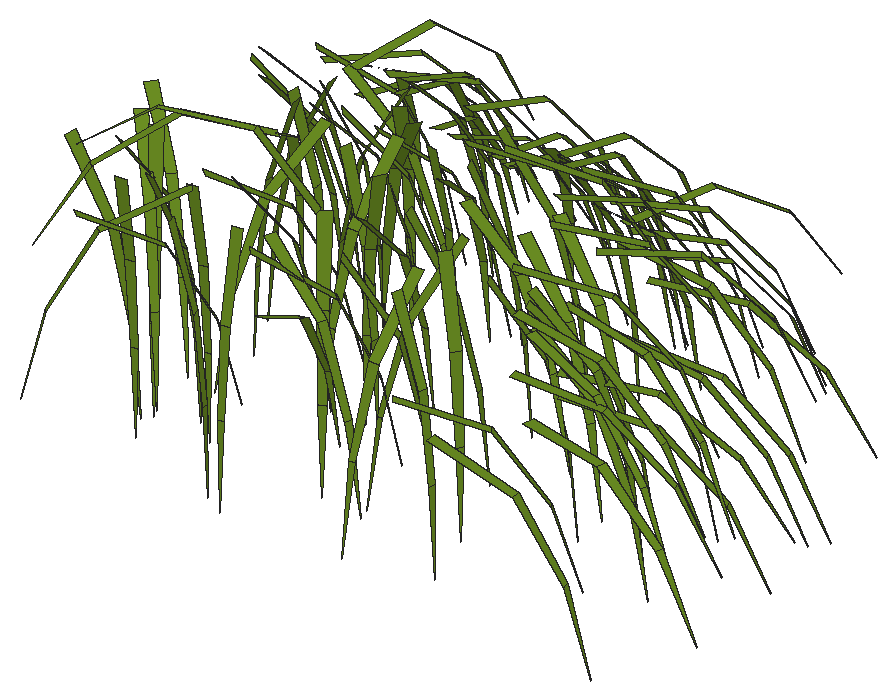
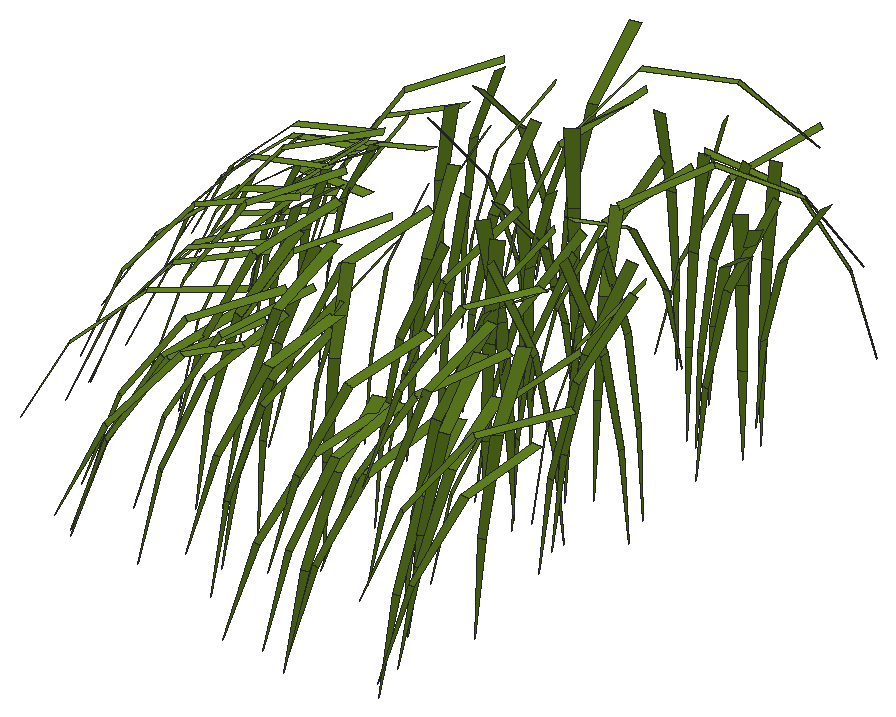
# SketchUp Ruby script. Lengths in inches.
U = 1.inch
M = Sketchup.active_model
def pt(a) = Geom::Point3d.new(a.map { |v| v * U })
def face(e, loops, mat)
  f = e.add_face(loops[0].map { |a| pt(a) })
  loops[1..].each { |l| e.add_face(l.map { |a| pt(a) }).erase! }
  f.material = f.back_material = mat if mat
  f
end
# faces: each face lists its corners as indices into pts; further lists are holes
def faces(e, pts, list, mat = nil) = list.each { |f| face(e, (f[0].is_a?(Array) ? f : [f]).map { |l| l.map { |i| pts[i] } }, mat) }
# xy, xz, yz: faces in a plane at the given z, y or x. An outline is a flat list of corners, or four numbers for a rectangle; further outlines are holes
def ring(l) = l.size == 4 ? [[l[0], l[1]], [l[2], l[1]], [l[2], l[3]], [l[0], l[3]]] : l.each_slice(2).to_a
def flat(e, list, mat, &to3) = list.each { |f| face(e, (f[0].is_a?(Array) ? f : [f]).map { |l| ring(l).map { |u, v| to3.(u, v) } }, mat) }
def xy(e, z, list, mat = nil) = flat(e, list, mat) { |x, y| [x, y, z] }
def xz(e, y, list, mat = nil) = flat(e, list, mat) { |x, z| [x, y, z] }
def yz(e, x, list, mat = nil) = flat(e, list, mat) { |y, z| [x, y, z] }
def lines(e, pts, list) = list.each { |a, b| e.add_line(pt(pts[a]), pt(pts[b])) }
# prism: a flat outline (further loops are holes) pulled along v
def prism(e, loops, v, mat = nil)
  f = face(e, loops, mat); d = Geom::Vector3d.new(v.map { |x| x * U })
  f.pushpull(f.normal.samedirection?(d) ? d.length : -d.length)
end
def box(e, o, s, mat = nil) = prism(e, [[o, [o[0] + s[0], o[1], o[2]], [o[0] + s[0], o[1] + s[1], o[2]], [o[0], o[1] + s[1], o[2]]]], [0, 0, s[2]], mat)
def at(x, y, z, deg = 0) = Geom::Transformation.translation(pt([x, y, z])) * Geom::Transformation.rotation(ORIGIN, Z_AXIS, deg.degrees)
def axes(o, x, y, z) = Geom::Transformation.new([*x, 0, *y, 0, *z, 0, *pt(o).to_a, 1])
def part(name) = M.definitions.add(name)
# library, detail: a bought-in or finely detailed component or shape, given as its bounding box
def library(name, o, s) = part(name).tap { |d| box(d.entities, o, s) }
def detail(e, o, s) = box(e.add_group.entities, o, s)
def put(e, d, t, mat = nil) = e.add_instance(d, t).tap { |i| i.material = mat if mat }
def group(e, t, mat = nil) = e.add_group.tap { |g| g.transformation = t; g.material = mat if mat }.entities
root = M.entities
M.materials.add("[0061_OliveDrab]").color = [107, 142, 35]
p = [[577.4,27.4,553.27],[577.52,27.24,553.27],[577.83,27.6,550.69],[579.25,28.79,553.23],[579.33,28.6,553.23],[580.26,29.11,550.83],
  [570.96,34.21,553.37],[571.13,34.15,553.37],[571.19,34.65,550.79],[579.23,19.85,553.375],[579.27,19.65,553.375],[579.96,19.875,550.85],
  [579.6875,25.77,553.27],[579.76,25.58,553.27],[580.75,26.09,550.9],[571.97,31.45,553.55],[572.16,31.44,553.55],[572.07,31.65,550.9375],
  [573.22,34.0625,553.41],[573.4,33.97,553.41],[573.58,34.56,550.86],[579.14,28.03,553.45],[579.23,27.84,553.45],[580.15,28.34,551.04],
  [575.1,33.91,553.47],[575.29,33.82,553.47],[575.58,34.74,551.03],[567,35.59,553.49],[567.2,35.54,553.49],[567.32,36.47,551.03],
  [567.17,35.74,553.4],[567.39,35.79,553.4],[567.04,36.88,551.03],[571.14,33.55,553.78],[571.34,33.49,553.78],[571.38,33.94,551.19],
  [574.95,34.1,553.68],[575.12,33.98,553.68],[575.56,34.78,551.22],[578.47,23.48,553.84],[578.44,23.27,553.84],[579.04,23.29,551.28],
  [575.6,24.49,553.95],[575.7,24.3125,553.95],[575.84,24.51,551.34],[577.35,25.26,553.89],[577.43,25.08,553.89],[577.78,25.34,551.3],
  [564.34,35.63,553.65],[564.53,35.68,553.65],[564.12,36.75,551.29],[580.33,22.28,553.7],[580.3,22.05,553.7],[581.66,22,551.45],
  [573.68,22.63,554.13],[573.5625,22.44,554.13],[573.72,22.47,551.51],[577.44,24.64,554.07],[577.46,24.42,554.07],[577.87,24.56,551.48],
  [573.36,31.89,554.05],[573.56,31.86,554.05],[573.52,32.32,551.47],[568.48,36.0625,553.85],[568.6875,36.03,553.85],[568.78,37.16,551.48],
  [574.38,20.58,554.19],[574.34,20.4,554.19],[574.48,20.46,551.57],[569.41,27.5,554.27],[569.59,27.48,554.27],[569.51,27.57,551.65],
  [565.81,33.08,554.16],[566.03,33.07,554.16],[565.9375,33.45,551.57],[567.48,36.03,553.97],[567.67,36.02,553.97],[567.59,37.07,551.56],
  [568.39,19.64,554.32],[568.2,19.62,554.32],[568.3,19.56,551.7],[567.52,20.01,554.35],[567.58,19.81,554.35],[567.64,19.93,551.73],
  [564.15,21.18,554.3],[564.36,21.21,554.3],[564.25,21.27,551.68],[569.86,21.9,554.3125],[569.68,21.78,554.3125],[569.81,21.78,551.6875],
  [565.78,22.125,554.32],[565.96,22.15,554.32],[565.86,22.23,551.69],[568.43,25.16,554.37],[568.54,25.33,554.37],[568.41,25.29,551.75],
  [571.83,27.46,554.33],[571.9,27.26,554.33],[572.02,27.42,551.71],[564.08,22.4,554.4],[563.9,22.27,554.4],[564.05,22.26,551.78],
  [568.84,25.24,554.4],[568.8,25.03,554.4],[568.93,25.11,551.78],[564.19,26.16,554.4],[564.17,26.35,554.4],[564.06,26.24,551.78],
  [566.01,26.86,554.39],[566,26.64,554.39],[566.14,26.75,551.77],[565.05,28.43,554.4375],[565.02,28.63,554.4375],[564.79,28.5,551.83],
  [566.62,29.15,554.41],[566.82,29.25,554.41],[566.66,29.32,551.79],[571.96,29.5,554.375],[571.99,29.29,554.375],[572.27,29.43,551.77],
  [568.84,30.63,554.45],[569.03,30.58,554.45],[568.99,30.82,551.84],[578.32,31.41,554.12],[578.41,31.23,554.12],[579.5,31.88,551.82],
  [565.1,22.52,554.5],[565.3,22.47,554.5],[565.24,22.625,551.88],[563.62,27.55,554.57],[563.6,27.76,554.57],[563.39,27.63,551.95],
  [565.98,28.8,554.54],[566.16,28.7,554.54],[566.14,28.87,551.92],[576.05,26.1,554.62],[575.98,25.91,554.62],[576.48,25.82,552.04],
  [568.96,32.62,554.52],[569.125,32.71,554.52],[568.78,33.125,551.95],[563.53,36.08,554.37],[563.71,36.06,554.37],[563.74,37.27,552.04],
  [571.77,21.73,554.67],[571.58,21.8125,554.67],[571.53,21.44,552.07],[572.8,24.43,554.67],[572.86,24.22,554.67],[573.11,24.4,552.06],
  [573.51,33.57,554.59],[573.68,33.44,554.59],[574.0625,34.11,552.08],[563.82,35.4,554.51],[564.02,35.4375,554.51],[563.73,36.47,552.12],
  [577.88,20.9,554.75],[578.01,20.73,554.75],[578.56,21.29,552.25],[564.0625,21.5,554.82],[564.04,21.28,554.82],[564.33,21.36,552.21],
  [573.03,21.91,554.8],[573.12,21.74,554.8],[573.3,21.9375,552.18],[563.625,24.19,554.82],[563.82,24.13,554.82],[563.81,24.43,552.21],
  [579.74,26.18,554.42],[579.84,25.98,554.42],[581.06,26.66,552.2],[566.32,28.59,554.8],[566.45,28.77,554.8],[566.1,28.87,552.2],
  [577.81,29.86,554.68],[577.86,29.65,554.68],[578.76,30,552.24],[565.29,32.36,554.75],[565.42,32.22,554.75],[565.74,32.65,552.18],
  [563.18,33.61,554.78],[563.38,33.68,554.78],[563.07,34.2,552.22],[572.875,19.28,554.86],[572.67,19.28,554.86],[572.77,18.87,552.27],
  [567.67,24.33,554.91],[567.85,24.22,554.91],[567.9,24.52,552.3],[574.87,33.66,554.8],[575.04,33.51,554.8],[575.5625,34.32,552.35],
  [568.39,24.06,555.02],[568.16,24.07,555.02],[568.25,23.72,552.41],[576.41,24.47,554.99],[576.33,24.26,554.99],[576.85,24.18,552.41],
  [568.27,28.53,555],[568.42,28.37,555],[568.625,28.71,552.41],[565.08,28.9,555.03],[565.18,28.74,555.03],[565.41,29.01,552.43],
  [563.47,30.6,555.04],[563.66,30.55,555.04],[563.65,30.92,552.4375],[564.42,34.52,554.84],[564.63,34.58,554.84],[564.3,35.35,552.35],
  [579.32,22.92,554.85],[579.28,22.73,554.85],[580.42,22.62,552.48],[579.86,23.48,554.84],[579.91,23.28,554.84],[581.14,23.65,552.55],
  [566.86,28.85,555.11],[567.0625,28.75,555.11],[567.12,29.13,552.51],[563.95,29.42,555.06],[564.16,29.41,555.06],[564.08,29.84,552.47],
  [564.625,21.71,555.24],[564.49,21.57,555.24],[564.86,21.35,552.65],[570.12,25.38,555.14],[570.3,25.39,555.14],[570.19,25.8,552.55],
  [579.28,25.28,555.12],[579.28,25.09,555.12],[580.3,25.2,552.7],[568.22,28.74,555.39],[568.21,28.54,555.39],[568.76,28.6,552.83],
  [569.48,28.53,555.42],[569.65,28.59,555.42],[569.4,29.02,552.84],[569.29,29.2,555.42],[569.46,29.1,555.42],[569.63,29.58,552.84],
  [572.125,20.09,555.49],[572.08,19.875,555.49],[572.58,19.88,552.91],[566.83,34.24,555.45],[567.02,34.13,555.45],[567.38,34.97,552.99],
  [568.08,34.97,555.43],[568.3,34.92,555.43],[568.38,35.86,552.98],[570.37,35.3,555.36],[570.58,35.29,555.36],[570.57,36.43,553],
  [571.47,22.08,555.65],[571.61,21.93,555.65],[571.91,22.37,553.08],[564.57,22.91,555.7],[564.44,22.74,555.7],[564.96,22.48,553.14],
  [571.16,33.31,555.59],[571.36,33.32,555.59],[571.21,34.11,553.09],[565.8,34.13,555.57],[565.98,34.125,555.57],[565.92,34.92,553.0625],
  [573.69,35.64,555.23],[573.89,35.5625,555.23],[574.31,36.97,553.05],[577.625,28.14,555.18],[577.74,27.87,555.18],[573.86,31.59,555.73],
  [574.06,31.52,555.73],[574.24,32.31,553.23],[564.79,34.91,555.55],[564.96,34.8,555.55],[565.47,35.8,553.18],[579.14,23.92,555.63],
  [579.16,23.72,555.63],[580.36,23.92,553.3],[567.84,24.96,555.9],[568,24.84,555.9],[568.29,25.38,553.35],[577.97,25.125,555.15],
  [578.07,24.86,555.15],[576.58,26.81,555.7],[576.75,26.6,555.7],[564.2,27.74,555.82],[564.36,27.83,555.82],[563.99,28.28,553.26],
  [576.12,29.54,555.84],[576.26,29.39,555.84],[576.77,30.07,553.35],[571.6,30.75,555.85],[571.79,30.64,555.85],[572.04,31.24,553.3],
  [577.82,19.65,555.58],[577.875,19.36,555.58],[566.42,22.49,555.98],[566.22,22.5,555.98],[566.29,21.87,553.43],[577.5625,27.42,555.45],
  [577.68,27.14,555.45],[573.43,30.77,555.96],[573.56,30.62,555.96],[574.05,31.15,553.44],[572.63,32.98,555.73],[572.89,32.85,555.73],
  [570.6,33.19,555.76],[570.85,33.11,555.76],[567.5,34,555.34],[567.8,34.07,555.34],[563.3125,18.85,556.04],[563.18,19.01,556.04],
  [562.75,18.52,553.5],[566.79,21.33,556.01],[566.93,21.21,556.01],[567.26,21.77,553.47],[577.56,30.24,555.91],[577.68,30.09,555.91],
  [578.39,30.83,553.49],[574.4,32.41,555.51],[574.67,32.29,555.51],[566.57,34.02,555.55],[566.85,33.95,555.55],[570.68,20.79,556.09],
  [570.87,20.83,556.09],[570.63,21.49,553.56],[575.38,24.23,556.16],[575.32,24.02,556.16],[576.03,23.92,553.64],[577.5,26.59,556.01],
  [577.61,26.41,556.01],[578.37,27,553.5625],[571.91,30.89,556.12],[572.1875,30.88,556.12],[578.28,22.58,555.32],[578.24,22.26,555.32],
  [573.96,32.78,555.73],[574.21,32.61,555.73],[564.8,33.91,555.58],[565.0625,33.99,555.58],[577.27,23.69,556.17],[577.23,23.4,556.17],
  [570.78,32.62,556.21],[571.07,32.53,556.21],[568.12,34.23,555.6875],[568.41,34.18,555.6875],[576.45,24.9,556.33],[576.56,24.65,556.33],
  [575.08,24.24,556.52],[575.22,23.99,556.52],[575.28,24.03,556.23],[567.4,34.22,555.87],[567.67,34.21,555.87],[573.45,22.82,556.74],
  [573.29,22.55,556.74],[576.5,24.61,556.51],[576.52,24.3,556.51],[576.52,30.57,555.84],[576.65,30.3125,555.84],[573.17,30.9,556.48],
  [573.45,30.86,556.48],[574.04,20.69,556.79],[573.98,20.4375,556.79],[565.74,32.22,556.64],[566.04,32.2,556.64],[568.4,19.85,556.94],
  [568.13,19.82,556.94],[567.27,19.98,556.96],[567.35,19.71,556.96],[564.13,20.99,556.92],[564.42,21.03,556.92],[569.8,22.08,556.93],
  [569.54,21.91,556.93],[565.78,21.89,556.93],[566.03,21.93,556.93],[571.43,27.35,556.93],[571.54,27.07,556.93],[569.34,27.29,556.88],
  [569.6,27.25,556.88],[563.95,22.66,557.01],[563.7,22.48,557.01],[568.62,24.98,556.98],[568.78,25.23,556.98],[568.55,25.34,557.01],
  [568.49,25.04,557.01],[577.83,25.35,556.02],[577.96,25.0625,556.02],[564.52,26.16,557.01],[564.49,26.43,557.01],[565.68,26.91,557],
  [565.68,26.6,557],[565.63,28.47,557],[565.59,28.75,557],[566.76,28.79,557.01],[567.04,28.94,557.01],[571.25,29.44,556.9],
  [571.29,29.15,556.9],[563.3,34.16,556.15],[563.5625,34.14,556.15],[564.97,22.15,557.1],[565.24,22.08,557.1],[565.75,28.49,557.13],
  [566,28.34,557.13],[568.66,30.09,557.02],[568.92,30.02,557.02],[569.46,31.63,556.9],[569.7,31.77,556.9],[564.09,33.68,556.47],
  [564.38,33.73,556.47],[575.08,26.54,557.02],[574.97,26.27,557.02],[564.14,27.55,557.14],[564.12,27.86,557.14],[572.59,32.45,556.77],
  [572.82,32.27,556.77],[572.13,22.43,557.18],[571.86,22.55,557.18],[572.19,24.29,557.22],[572.28,24,557.22],[576.18,29.49,556.71],
  [576.25,29.19,556.71],[564.46,31.63,557.13],[564.65,31.43,557.13],[576.67,20.01,556.91],[576.85,19.77,556.91],[563.41,21.61,557.36],
  [563.375,21.3,557.36],[572.45,21.67,557.35],[572.57,21.42,557.35],[577.54,23.3,556.74],[577.49,23.02,556.74],[577.9,23.11,556.54],
  [577.96,22.83,556.54],[563.38,23.57,557.36],[563.66,23.48,557.36],[566.91,28.14,557.32],[567.09,28.4,557.32],[573.74,32.37,556.79],
  [573.98,32.17,556.79],[563.57,32.45,557.1],[563.86,32.56,557.1],[564.79,33.06,556.99],[565.09,33.14,556.99],[572.92,20.16,557.33],
  [572.62,20.16,557.33],[567.29,23.74,557.44],[567.56,23.6,557.44],[568.49,24.85,557.52],[568.17,24.87,557.52],[575.39,24.9,557.37],
  [575.28,24.62,557.37],[575.78,24.45,556.24],[567.63,28,557.49],[567.84,27.77,557.49],[564.4,28.49,557.53],[564.55,28.27,557.53],
  [563.24,29.81,557.53],[563.5,29.74,557.53],[575.57,24.19,555.68],[575.7,23.86,555.68],[570.12,24.49,557.61],[570.38,24.5,557.61],
  [577.5,25.29,557.06],[577.51,25.03,557.06],[566.46,28.12,557.6],[566.75,27.98,557.6],[563.86,28.55,557.53],[564.17,28.53,557.53],
  [563.99,22.39,557.69],[563.8,22.19,557.69],[575.29,27.17,555.91],[575.43,26.85,555.91],[572.86,33.57,556.62],[573.13,33.46,556.62],
  [575.6875,22.93,555.53],[575.64,22.54,555.53],[567.98,31.6,556.27],[568.35,31.68,556.27],[569.8,27.53,557.83],[570.04,27.61,557.83],
  [568.72,28.32,557.83],[568.96,28.17,557.83],[567.09,28.86,557.76],[567.07,28.58,557.76],[567.68,33.32,557.43],[567.99,33.25,557.43],
  [570.17,33.43,557.19],[570.47,33.41,557.19],[571.11,20.35,557.9],[571.04,20.06,557.9],[575.3,26.51,556.43],[575.44,26.17,556.43],
  [573.375,30.15,556.37],[573.72,30,556.37],[565.96,32.86,557.51],[566.23,32.7,557.51],[575.43,19.26,556.58],[575.49,18.9,556.58],
  [577.23,23.82,557.43],[577.26,23.53,557.43],[565.45,31.55,556.51],[565.77,31.64,556.51],[565.95,31.64,556.47],[566.29,31.56,556.47],
  [571.2,31.77,557.72],[571.48,31.79,557.72],[565.7,32.625,557.71],[565.96,32.62,557.71],[563.73,33.33,557.36],[563.97,33.17,557.36],
  [570.63,21.33,558.03],[570.84,21.11,558.03],[563.67,23.66,558.05],[563.49,23.43,558.05],[574.97,25.59,557.37],[575.17,25.33,557.37],
  [573.29,30.16,557.86],[573.5625,30.0625,557.86],[572.49,30.75,556.48],[572.78,30.54,556.48],[571.6,30.98,557.09],[571.91,30.83,557.09],
  [567.64,31.69,556.17],[567.99,31.63,556.17],[565.96,33.51,558],[566.15,33.47,558],[566.3,34.66,555.67],[564.77,26.68,558.16],
  [565,26.82,558.16],[574.99,28.44,557.94],[575.2,28.23,557.94],[574.18,29.45,556.21],[574.33,29.14,556.21],[570.87,29.68,558.125],
  [571.14,29.51,558.125],[569.93,31.16,557.29],[570.23,31.07,557.29],[567.0625,23.99,558.21],[567.28,23.82,558.21],[576.15,29.06,557.78],
  [576.32,28.85,557.78],[567.3125,31.63,556.32],[567.65,31.63,556.32],[564.34,19.66,558.32],[564.16,19.88,558.32],[565.94,20.34,558.29],
  [566.15,20.17,558.29],[566.54,23.76,558.27],[566.25,23.78,558.27],[575.4375,24.3,556.27],[575.6,23.94,556.27],[576.02,25.74,558],
  [576.17,25.5,558],[572.3,29.91,558.16],[572.48,29.68,558.16],[570.92,19.45,558.33],[571.19,19.51,558.33],[571.84,29.4,558.28],
  [572.18,29.39,558.28],[575.03,24.04,557.49],[574.98,23.69,557.49],[574.04,24.6875,558.37],[573.94,24.38,558.37],[570.1,30.6875,557.85],
  [570.45,30.57,557.85],[563.02,31.59,556.6],[563.34,31.56,556.6],[574.6,24.11,558.01],[574.74,23.79,558.01],[571.91,31.14,556.29],
  [572.24,31.02,556.29],[575.35,22.61,556.92],[575.43,22.27,556.92],[573.78,23.55,558.6875],[573.96,23.24,558.6875],[574.51,24.48,558.22],
  [574.54,24.1,558.22],[572.84,28.86,558.1],[573.18,28.81,558.1],[564.51,31.22,557.31],[564.86,31.29,557.31],[565.625,30.33,558.47],
  [566,30.32,558.47],[572.84,23.21,559.26],[572.65,22.89,559.26],[575.0625,23.79,557.46],[575,23.45,557.46],[573.74,28.9,557.48],
  [573.83,28.53,557.48],[573.04,20.94,559.21],[572.97,20.625,559.21],[572.07,30.42,557.35],[572.375,30.17,557.35],[571.07,30.57,557.81],
  [571.36,30.35,557.81],[574.7,18.51,557.79],[574.92,18.23,557.79],[568.36,20.42,559.5],[568.03,20.38,559.5],[564.16,20.53,559.5],
  [564.51,20.58,559.5],[565.82,21.36,559.5],[565.95,21.38,559.5],[566.14,21.41,559.5],[569.54,22.54,559.5],[569.25,22.35,559.5],
  [569.22,22.33,559.5],[569.23,26.72,559.45],[569.54,26.68,559.45],[570.45,27,559.34],[570.59,26.66,559.34],[569.69,29.27,559.01],
  [569.74,28.91,559.01],[570.46,29.78,558.47],[570.75,29.94,558.47],[566.62,19.84,559.5],[566.71,19.5,559.5],[563.04,21.03,559.18],
  [562.875,21.16,559.18],[562.02,19.95,557.02],[563.49,23.36,559.5],[563.18,23.13,559.5],[569.23,24.5625,559.5],[569.42,24.86,559.5],
  [567.74,25.53,559.5],[567.67,25.17,559.5],[565.34,26.22,559.5],[565.3,26.55,559.5],[573.16,27.36,558.61],[573.02,27.03,558.61],
  [564.89,26.95,559.5],[564.89,26.57,559.5],[567.22,27.82,559.4],[567.57,28,559.4],[566.93,28.61,559.27],[566.88,28.96,559.27],
  [568.28,28.74,559.24],[568.61,28.66,559.24],[565.42,30.73,558.02],[565.79,30.83,558.02],[564.67,21.13,559.5],[565.01,21.05,559.5],
  [574.9375,25.28,557.6],[574.94,24.96,557.6],[565.15,27.52,559.5],[565.46,27.34,559.5],[565.35,27.625,559.47],[565.3125,28.01,559.47],
  [562.88,30.18,558.65],[563.12,29.93,558.65],[564.34,30.32,558.43],[564.7,30.45,558.43],[572.82,23.89,559.24],[572.5,24.03,559.24],
  [570.94,23.96,559.5],[571.05,23.59,559.5],[569.92,30.86,557.62],[570.29,30.83,557.62],[572.94,21.95,559.26],[572.58,21.95,559.26],
  [571.09,21.03,559.5],[571.24,20.73,559.5],[568.17,27.25,559.45],[568.38,27.57,559.45],[561.9,21.79,559.5],[561.87,21.42,559.5],
  [562.9,22.14,559.5],[563.24,22.03,559.5],[566.47,22.34,559.5],[566.8,22.16,559.5],[574.67,23.65,557.98],[574.7,23.3,557.98],
  [573.375,25.7,558.85],[573.24,25.35,558.85],[567.11,30.82,558.02],[567.49,30.74,558.02],[562.3,31.14,557.62],[562.59,30.95,557.62],
  [568.63,26.56,559.5],[568.25,26.58,559.5],[566.37,26.87,559.5],[566.63,26.59,559.5],[563.75,26.82,559.5],[564.12,26.8,559.5],
  [562.95,27.54,559.5],[563.125,27.28,559.5],[562.78,28.05,559.43],[563.1,27.97,559.43],[564.65,30.71,558.26],[564.98,30.52,558.26],
  [570.17,22.67,559.5],[570.49,22.68,559.5],[565.66,26.5,559.5],[566.02,26.33,559.5],[562.65,23.74,559.5],[562.42,23.5,559.5],
  [571.3,29.26,558.48],[571.65,29.28,558.48],[565.58,30.15,558.59],[565.9,30.14,558.59],[570.47,25.5625,559.43],[570.77,25.67,559.43],
  [567.66,26.6,559.5],[567.96,26.42,559.5],[574.15,27.36,557.94],[574.37,27.1,557.94],[564.94,29.04,559.26],[564.92,28.71,559.26],
  [564.95,29.04,559.26],[569.08,20.83,559.5],[569.01,20.47,559.5],[573.21,26.65,558.69],[573.47,26.4,558.69],[572.39,27.83,558.66],
  [572.73,27.71,558.66],[569.06,19.83,559.5],[569.31,19.57,559.5],[561.96,25.03,559.5],[561.74,24.74,559.5],[573.83,24.45,558.64],
  [574.01,24.15,558.64],[565.49,31.5,559.625],[565.77,31.44,559.625],[569.59,27.71,559.31],[569.92,27.51,559.31],[565.66,22.18,559.5],
  [565.93,21.98,559.5],[565.89,24.72,559.5],[566,24.79,559.5],[566.17,24.89,559.5],[570.39,28.39,559.14],[570.62,28.11,559.14],
  [571.37,17.14,559.5],[571.71,17.21,559.5],[564.46,18.54,559.5],[564.72,18.34,559.5],[566.16,21.13,559.5],[565.93,21.41,559.5],
  [566.7,26.07,559.5],[566.35,26.09,559.5],[571.71,25.43,559.34],[571.6,25.06,559.34],[564.55,22.8,560.4],[564.3125,22.99,560.4],
  [564.93,28.97,559.25],[565.27,28.9,559.25],[569.31,22.16,559.5],[569.2,22.5,559.5],[567.64,21.9375,561.54],[567.73,21.66,561.54],
  [566.14,24.6875,559.5],[565.85,24.92,559.5],[565.23,20.87,561.67],[565.17,21.0625,561.67],[563.15,20.28,560.18]]
faces(root,p,[[0,1,2],[3,4,5],[6,7,8],[9,10,11],[12,13,14],[15,16,17],[18,19,20],[21,22,23],
  [24,25,26],[27,28,29],[30,31,32],[33,34,35],[36,37,38],[39,40,41],[42,43,44],[45,46,47],
  [48,49,50],[51,52,53],[54,55,56],[57,58,59],[60,61,62],[63,64,65],[66,67,68],[69,70,71],
  [72,73,74],[75,76,77],[78,79,80],[81,82,83],[84,85,86],[87,88,89],[90,91,92],[93,94,95],
  [96,97,98],[99,100,101],[102,103,104],[105,106,107],[108,109,110],[111,112,113],[114,115,116],[117,118,119],
  [120,121,122],[123,124,125],[126,127,128],[129,130,131],[132,133,134],[135,136,137],[138,139,140],[141,142,143],
  [144,145,146],[147,148,149],[150,151,152],[153,154,155],[156,157,158],[159,160,161],[162,163,164],[165,166,167],
  [168,169,170],[171,172,173],[174,175,176],[177,178,179],[180,181,182],[183,184,185],[186,187,188],[189,190,191],
  [192,193,194],[195,196,197],[198,199,200],[201,202,203],[204,205,206],[207,208,209],[210,211,212],[213,214,215],
  [216,217,218],[219,220,221],[222,223,224],[225,226,227],[228,229,230],[231,232,233],[234,235,236],[237,238,239],
  [240,241,242],[243,244,245],[246,247,248],[249,250,251],[252,253,254],[255,256,257],[258,259,260],[261,262,263],
  [264,265,266],[267,268,4,3],[269,270,271],[272,273,274],[275,276,277],[278,279,280],[281,282,13,12],[283,284,1,0],
  [285,286,287],[288,289,290],[291,292,293],[294,295,10,9],[296,297,298],[299,300,22,21],[301,302,303],[304,305,19,18],
  [306,307,7,6],[308,309,31,30],[310,311,312],[313,314,315],[316,317,318],[319,320,25,24],[321,322,28,27],[323,324,325],
  [326,327,328],[329,330,331],[332,333,16,15],[334,335,52,51],[336,337,37,36],[338,339,49,48],[340,341,40,39],[342,343,34,33],
  [344,345,64,63],[346,347,46,45],[348,349,350,43,42],[351,352,76,75],[353,354,55,54],[355,356,58,57],[357,358,124,123],[359,360,61,60],
  [361,362,67,66],[363,364,73,72],[365,366,79,78],[367,368,82,81],[369,370,85,84],[371,372,88,87],[373,374,91,90],[375,376,97,96],
  [377,378,70,69],[379,380,100,99],[381,382,94,93],[383,384,103,102],[385,386,169,168],[387,388,106,105],[389,390,109,108],[391,392,112,111],
  [393,394,115,114],[395,396,118,117],[397,398,142,141],[399,400,127,126],[401,402,133,132],[403,404,121,120],[405,406,139,138],[407,408,154,153],
  [409,410,136,135],[411,412,130,129],[413,414,151,150],[415,416,145,144],[417,418,148,147],[419,420,175,174],[421,422,178,177],[423,424,157,156],
  [425,426,160,159],[427,428,163,162],[429,430,211,210],[431,432,214,213],[433,434,166,165],[435,436,172,171],[437,438,190,189],[439,440,181,180],
  [441,442,208,207],[443,444,184,183],[445,446,187,186],[447,448,193,192],[449,450,451,196,195],[452,453,199,198],[454,455,202,201],[456,457,205,204],
  [458,459,282,281],[460,461,226,225],[462,463,229,228],[464,465,217,216],[466,467,220,219],[468,469,223,222],[470,471,268,267],[472,473,265,264],
  [474,475,335,334],[476,477,309,308],[478,479,235,234],[480,481,238,237],[482,483,232,231],[484,485,247,246],[486,487,250,249],[488,489,241,240],
  [490,491,300,299],[492,493,320,319],[494,495,244,243],[496,497,295,294],[498,499,276,275],[500,501,339,338],[502,503,322,321],[504,505,259,258],
  [506,507,262,261],[508,509,273,272],[510,511,253,252],[512,513,256,255],[514,515,284,283],[516,517,270,269],[518,519,337,336],[520,521,305,304],
  [522,523,345,344],[524,525,526],[527,528,286,285],[529,530,289,288],[531,532,358,357],[533,534,292,291],[535,536,307,306],[537,538,279,278],
  [539,540,317,316],[541,542,352,351],[543,544,311,310],[545,546,314,313],[547,548,297,296],[549,550,386,385,451],[551,552,330,329],[553,554,302,301],
  [555,556,324,323],[557,558,333,332],[559,560,341,340],[561,562,350,327,326],[563,564,343,342],[565,566,398,397],[567,568,347,346],[569,570,473,472],
  [571,572,432,431],[573,574,349,348],[575,576,356,355],[577,578,360,359],[579,580,408,407],[581,582,364,363],[583,584,354,353],[585,586,430,429],
  [587,588,420,419],[589,590,362,361],[591,592,438,437],[593,594,414,413],[595,596,424,423],[597,598,366,365],[599,600,370,369],[601,602,603,374,373],
  [604,605,606,372,371],[607,608,378,377],[609,610,376,375],[611,612,396,395],[613,614,406,405],[615,616,368,367],[617,618,619],[620,621,380,379],
  [622,623,382,381],[624,625,384,383],[626,627,388,387],[628,629,410,409],[630,631,390,389],[632,633,394,393],[634,635,392,391],[636,637,404,403],
  [638,639,442,441],[640,641,400,399],[642,643,463,462],[644,645,402,401],[646,647,412,411],[648,649,422,421],[650,651,440,439],[652,653,416,415],
  [654,655,418,417],[656,657,487,486],[658,659,444,443],[660,661,428,427],[662,663,436,435],[664,665,426,425],[666,667,434,433],[668,669,446,445],
  [670,671,499,498],[672,673,450,449],[674,675,485,484],[676,677,509,508],[678,679,448,447],[680,681,453,452],[682,683,467,466],[684,685,455,454],
  [686,687,457,456],[688,689,495,494],[690,691,461,460],[692,693,465,464],[694,695,469,468],[696,697,505,504],[698,699,507,506],[700,701,479,478],
  [702,703,481,480],[704,705,540,539],[706,707,483,482,708],[709,710,489,488],[711,712,530,529],[713,714,517,516],[715,716,511,510],[717,718,513,512],
  [719,720,552,551],[721,722,525,524],[723,724,534,533],[725,726,538,537],[727,728,729,528,527],[730,731,554,553],[732,733,556,555],[734,735,546,545],
  [736,602,737,544,543],[738,739,548,547],[740,741,562,561],[742,743,618,617],[744,745,722,721,708],[746,605,747,748,749],[750,728,751,743,742],[752,753,754],
  [749,748,753,752]],"[0061_OliveDrab]")
